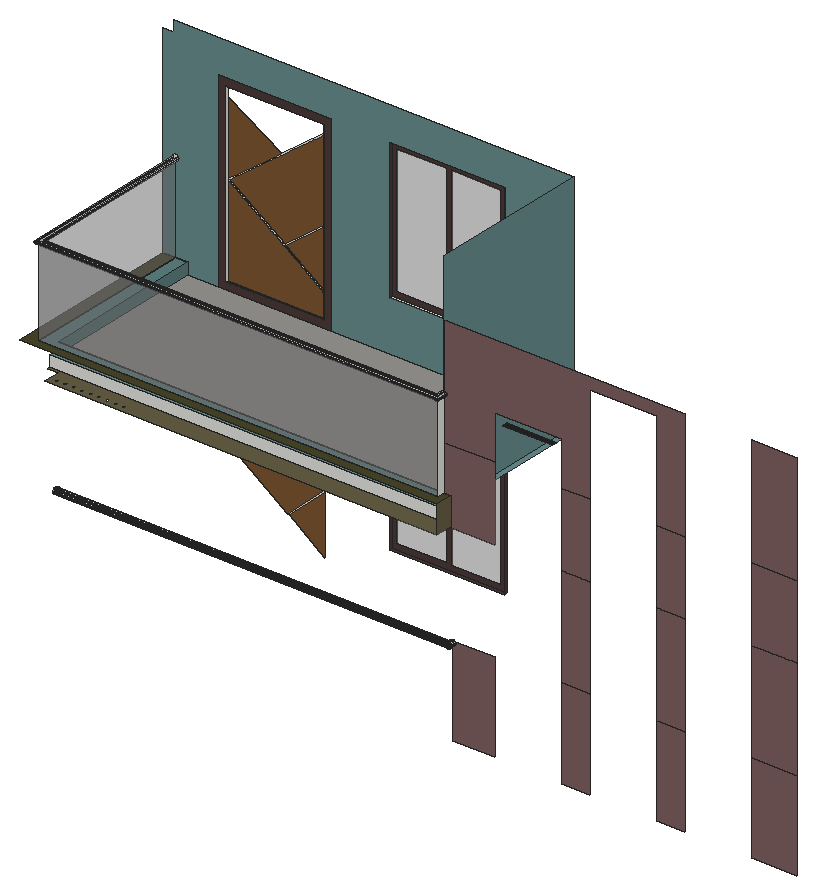
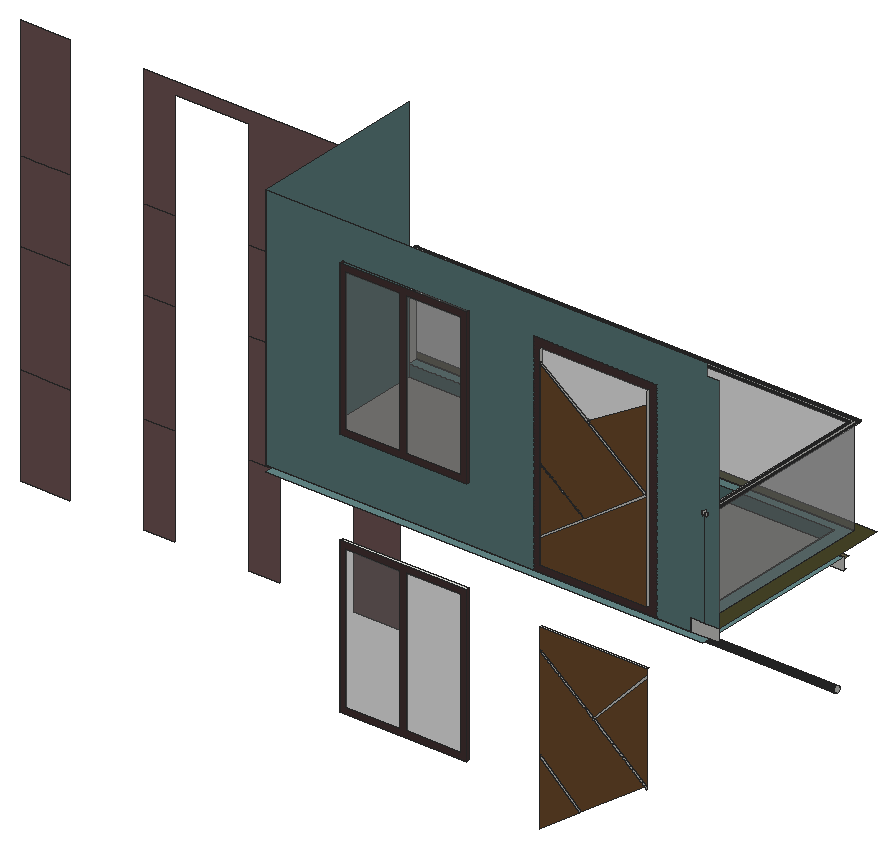
# SketchUp Ruby script. Lengths in inches.
U = 1.inch
M = Sketchup.active_model
def pt(a) = Geom::Point3d.new(a.map { |v| v * U })
def face(e, loops, mat)
  f = e.add_face(loops[0].map { |a| pt(a) })
  loops[1..].each { |l| e.add_face(l.map { |a| pt(a) }).erase! }
  f.material = f.back_material = mat if mat
  f
end
# faces: each face lists its corners as indices into pts; further lists are holes
def faces(e, pts, list, mat = nil) = list.each { |f| face(e, (f[0].is_a?(Array) ? f : [f]).map { |l| l.map { |i| pts[i] } }, mat) }
# xy, xz, yz: faces in a plane at the given z, y or x. An outline is a flat list of corners, or four numbers for a rectangle; further outlines are holes
def ring(l) = l.size == 4 ? [[l[0], l[1]], [l[2], l[1]], [l[2], l[3]], [l[0], l[3]]] : l.each_slice(2).to_a
def flat(e, list, mat, &to3) = list.each { |f| face(e, (f[0].is_a?(Array) ? f : [f]).map { |l| ring(l).map { |u, v| to3.(u, v) } }, mat) }
def xy(e, z, list, mat = nil) = flat(e, list, mat) { |x, y| [x, y, z] }
def xz(e, y, list, mat = nil) = flat(e, list, mat) { |x, z| [x, y, z] }
def yz(e, x, list, mat = nil) = flat(e, list, mat) { |y, z| [x, y, z] }
def lines(e, pts, list) = list.each { |a, b| e.add_line(pt(pts[a]), pt(pts[b])) }
# prism: a flat outline (further loops are holes) pulled along v
def prism(e, loops, v, mat = nil)
  f = face(e, loops, mat); d = Geom::Vector3d.new(v.map { |x| x * U })
  f.pushpull(f.normal.samedirection?(d) ? d.length : -d.length)
end
def box(e, o, s, mat = nil) = prism(e, [[o, [o[0] + s[0], o[1], o[2]], [o[0] + s[0], o[1] + s[1], o[2]], [o[0], o[1] + s[1], o[2]]]], [0, 0, s[2]], mat)
def at(x, y, z, deg = 0) = Geom::Transformation.translation(pt([x, y, z])) * Geom::Transformation.rotation(ORIGIN, Z_AXIS, deg.degrees)
def axes(o, x, y, z) = Geom::Transformation.new([*x, 0, *y, 0, *z, 0, *pt(o).to_a, 1])
def part(name) = M.definitions.add(name)
# library, detail: a bought-in or finely detailed component or shape, given as its bounding box
def library(name, o, s) = part(name).tap { |d| box(d.entities, o, s) }
def detail(e, o, s) = box(e.add_group.entities, o, s)
def put(e, d, t, mat = nil) = e.add_instance(d, t).tap { |i| i.material = mat if mat }
def group(e, t, mat = nil) = e.add_group.tap { |g| g.transformation = t; g.material = mat if mat }.entities
root = M.entities
M.materials.add("[0057_DarkKhaki]").color = [71, 69, 40]
M.materials.add("[0089_PaleTurquoise]").color = [103, 140, 140]
M.materials.add("[0089_PaleTurquoise]2").color = [93, 127, 127]
M.materials.add("[0119_RosyBrown]").color = [127, 96, 96]
M.materials.add("[0119_RosyBrown]1").color = [76, 58, 58]
M.materials.add("[0136_Charcoal]").color = [35, 35, 35]
M.materials.add("[Granite Light Gray]").color = [149, 148, 144]
M.materials.add("[Translucent Glass Gray]").color = [130, 130, 130]
M.materials["[Translucent Glass Gray]"].alpha = 0.5
M.materials.add("[Translucent Glass Gray]1").color = [128, 128, 128]
M.materials["[Translucent Glass Gray]1"].alpha = 0.5
M.materials.add("[Wood Floor]").color = [124, 84, 49]
M.materials.add("[Wood Lumber ButtJoined]").color = [102, 94, 69]
xy(root,619.5,[[726,546,973.25,552]],"[0119_RosyBrown]1")
xy(root,903.9,[[375.6,546,584.4,551]])
xy(root,919.5,[[726,546,973.25,552]])
xy(root,960,[[[294,162,294,198,270,198,270,204,1122,204,1122,198,1135.625,198,1135.625,162],[308.5625,171.77,309.6,171.91,310.5625,172.31,311.39,172.94,312.03,173.77,312.43,174.74,312.5625,175.77,312.43,176.81,312.03,177.77,311.39,178.6,310.5625,179.24,309.6,179.64,308.5625,179.77,307.53,179.64,306.5625,179.24,305.73,178.6,305.1,177.77,304.7,176.81,304.5625,175.77,304.7,174.74,305.1,173.77,305.73,172.94,306.5625,172.31,307.53,171.91],[326.5625,171.77,327.6,171.91,328.5625,172.31,329.39,172.94,330.03,173.77,330.43,174.74,330.5625,175.77,330.43,176.81,330.03,177.77,329.39,178.6,328.5625,179.24,327.6,179.64,326.5625,179.77,325.53,179.64,324.5625,179.24,323.73,178.6,323.1,177.77,322.7,176.81,322.5625,175.77,322.7,174.74,323.1,173.77,323.73,172.94,324.5625,172.31,325.53,171.91],[344.5625,171.77,345.6,171.91,346.5625,172.31,347.39,172.94,348.03,173.77,348.43,174.74,348.5625,175.77,348.43,176.81,348.03,177.77,347.39,178.6,346.5625,179.24,345.6,179.64,344.5625,179.77,343.53,179.64,342.5625,179.24,341.73,178.6,341.1,177.77,340.7,176.81,340.5625,175.77,340.7,174.74,341.1,173.77,341.73,172.94,342.5625,172.31,343.53,171.91],[362.5625,171.77,363.6,171.91,364.5625,172.31,365.39,172.94,366.03,173.77,366.43,174.74,366.5625,175.77,366.43,176.81,366.03,177.77,365.39,178.6,364.5625,179.24,363.6,179.64,362.5625,179.77,361.53,179.64,360.5625,179.24,359.73,178.6,359.1,177.77,358.7,176.81,358.5625,175.77,358.7,174.74,359.1,173.77,359.73,172.94,360.5625,172.31,361.53,171.91],[380.5625,171.77,381.6,171.91,382.5625,172.31,383.39,172.94,384.03,173.77,384.43,174.74,384.5625,175.77,384.43,176.81,384.03,177.77,383.39,178.6,382.5625,179.24,381.6,179.64,380.5625,179.77,379.53,179.64,378.5625,179.24,377.73,178.6,377.1,177.77,376.7,176.81,376.5625,175.77,376.7,174.74,377.1,173.77,377.73,172.94,378.5625,172.31,379.53,171.91],[398.5625,171.77,399.6,171.91,400.5625,172.31,401.39,172.94,402.03,173.77,402.43,174.74,402.5625,175.77,402.43,176.81,402.03,177.77,401.39,178.6,400.5625,179.24,399.6,179.64,398.5625,179.77,397.53,179.64,396.5625,179.24,395.73,178.6,395.1,177.77,394.7,176.81,394.5625,175.77,394.7,174.74,395.1,173.77,395.73,172.94,396.5625,172.31,397.53,171.91],[416.5625,171.77,417.6,171.91,418.5625,172.31,419.39,172.94,420.03,173.77,420.43,174.74,420.5625,175.77,420.43,176.81,420.03,177.77,419.39,178.6,418.5625,179.24,417.6,179.64,416.5625,179.77,415.53,179.64,414.5625,179.24,413.73,178.6,413.1,177.77,412.7,176.81,412.5625,175.77,412.7,174.74,413.1,173.77,413.73,172.94,414.5625,172.31,415.53,171.91],[434.5625,171.77,435.6,171.91,436.5625,172.31,437.39,172.94,438.03,173.77,438.43,174.74,438.5625,175.77,438.43,176.81,438.03,177.77,437.39,178.6,436.5625,179.24,435.6,179.64,434.5625,179.77,433.53,179.64,432.5625,179.24,431.73,178.6,431.1,177.77,430.7,176.81,430.5625,175.77,430.7,174.74,431.1,173.77,431.73,172.94,432.5625,172.31,433.53,171.91],[452.5625,171.77,453.6,171.91,454.5625,172.31,455.39,172.94,456.03,173.77,456.43,174.74,456.5625,175.77,456.43,176.81,456.03,177.77,455.39,178.6,454.5625,179.24,453.6,179.64,452.5625,179.77,451.53,179.64,450.5625,179.24,449.73,178.6,449.1,177.77,448.7,176.81,448.5625,175.77,448.7,174.74,449.1,173.77,449.73,172.94,450.5625,172.31,451.53,171.91]]],"[Wood Lumber ButtJoined]")
xy(root,984,[[382.18,289.15,379.08,289.56,376.18,290.76,373.7,292.66,371.79,295.15,370.59,298.04,370.18,301.15,370.59,304.26,371.79,307.15,373.7,309.63,376.18,311.54,379.08,312.74,382.18,313.15,385.29,312.74,388.18,311.54,390.67,309.63,392.58,307.15,393.77,304.26,394.18,301.15,393.77,298.04,392.58,295.15,390.67,292.66,388.18,290.76,385.29,289.56],[706.18,289.15,703.08,289.56,700.18,290.76,697.7,292.66,695.79,295.15,694.59,298.04,694.18,301.15,694.59,304.26,695.79,307.15,697.7,309.63,700.18,311.54,703.08,312.74,706.18,313.15,709.29,312.74,712.18,311.54,714.67,309.63,716.58,307.15,717.77,304.26,718.18,301.15,717.77,298.04,716.58,295.15,714.67,292.66,712.18,290.76,709.29,289.56],[1030.18,289.15,1027.08,289.56,1024.18,290.76,1021.7,292.66,1019.79,295.15,1018.59,298.04,1018.18,301.15,1018.59,304.26,1019.79,307.15,1021.7,309.63,1024.18,311.54,1027.08,312.74,1030.18,313.15,1033.29,312.74,1036.18,311.54,1038.67,309.63,1040.58,307.15,1041.77,304.26,1042.18,301.15,1041.77,298.04,1040.58,295.15,1038.67,292.66,1036.18,290.76,1033.29,289.56],[382.18,409.15,379.08,409.56,376.18,410.76,373.7,412.66,371.79,415.15,370.59,418.04,370.18,421.15,370.59,424.26,371.79,427.15,373.7,429.63,376.18,431.54,379.08,432.74,382.18,433.15,385.29,432.74,388.18,431.54,390.67,429.63,392.58,427.15,393.77,424.26,394.18,421.15,393.77,418.04,392.58,415.15,390.67,412.66,388.18,410.76,385.29,409.56],[706.18,409.15,703.08,409.56,700.18,410.76,697.7,412.66,695.79,415.15,694.59,418.04,694.18,421.15,694.59,424.26,695.79,427.15,697.7,429.63,700.18,431.54,703.08,432.74,706.18,433.15,709.29,432.74,712.18,431.54,714.67,429.63,716.58,427.15,717.77,424.26,718.18,421.15,717.77,418.04,716.58,415.15,714.67,412.66,712.18,410.76,709.29,409.56],
  [1030.18,409.15,1027.08,409.56,1024.18,410.76,1021.7,412.66,1019.79,415.15,1018.59,418.04,1018.18,421.15,1018.59,424.26,1019.79,427.15,1021.7,429.63,1024.18,431.54,1027.08,432.74,1030.18,433.15,1033.29,432.74,1036.18,431.54,1038.67,429.63,1040.58,427.15,1041.77,424.26,1042.18,421.15,1041.77,418.04,1040.58,415.15,1038.67,412.66,1036.18,410.76,1033.29,409.56]])
xy(root,984,[[[270,204,1122,546],[382.18,409.15,385.29,409.56,388.18,410.76,390.67,412.66,392.58,415.15,393.77,418.04,394.18,421.15,393.77,424.26,392.58,427.15,390.67,429.63,388.18,431.54,385.29,432.74,382.18,433.15,379.08,432.74,376.18,431.54,373.7,429.63,371.79,427.15,370.59,424.26,370.18,421.15,370.59,418.04,371.79,415.15,373.7,412.66,376.18,410.76,379.08,409.56],[382.18,289.15,385.29,289.56,388.18,290.76,390.67,292.66,392.58,295.15,393.77,298.04,394.18,301.15,393.77,304.26,392.58,307.15,390.67,309.63,388.18,311.54,385.29,312.74,382.18,313.15,379.08,312.74,376.18,311.54,373.7,309.63,371.79,307.15,370.59,304.26,370.18,301.15,370.59,298.04,371.79,295.15,373.7,292.66,376.18,290.76,379.08,289.56],[706.18,409.15,709.29,409.56,712.18,410.76,714.67,412.66,716.58,415.15,717.77,418.04,718.18,421.15,717.77,424.26,716.58,427.15,714.67,429.63,712.18,431.54,709.29,432.74,706.18,433.15,703.08,432.74,700.18,431.54,697.7,429.63,695.79,427.15,694.59,424.26,694.18,421.15,694.59,418.04,695.79,415.15,697.7,412.66,700.18,410.76,703.08,409.56],[1030.18,409.15,1033.29,409.56,1036.18,410.76,1038.67,412.66,1040.58,415.15,1041.77,418.04,1042.18,421.15,1041.77,424.26,1040.58,427.15,1038.67,429.63,1036.18,431.54,1033.29,432.74,1030.18,433.15,1027.08,432.74,1024.18,431.54,1021.7,429.63,1019.79,427.15,1018.59,424.26,1018.18,421.15,1018.59,418.04,1019.79,415.15,1021.7,412.66,1024.18,410.76,1027.08,409.56],[706.18,289.15,709.29,289.56,712.18,290.76,714.67,292.66,716.58,295.15,717.77,298.04,718.18,301.15,717.77,304.26,716.58,307.15,714.67,309.63,712.18,311.54,709.29,312.74,706.18,313.15,703.08,312.74,700.18,311.54,697.7,309.63,695.79,307.15,694.59,304.26,694.18,301.15,694.59,298.04,695.79,295.15,697.7,292.66,700.18,290.76,703.08,289.56],[1030.18,289.15,1033.29,289.56,1036.18,290.76,1038.67,292.66,1040.58,295.15,1041.77,298.04,1042.18,301.15,1041.77,304.26,1040.58,307.15,1038.67,309.63,1036.18,311.54,1033.29,312.74,1030.18,313.15,1027.08,312.74,1024.18,311.54,1021.7,309.63,1019.79,307.15,1018.59,304.26,1018.18,301.15,1018.59,298.04,1019.79,295.15,1021.7,292.66,1024.18,290.76,1027.08,289.56]]],"[0089_PaleTurquoise]")
xy(root,996,[[294,198,1122,546]],"[Granite Light Gray]")
xy(root,1011.6,[[375.6,546,584.4,551]])
xy(root,1020,[[240,162,1135.625,162,1135.625,198,1122,198,1122,180,267,180,267,546,240,546]],"[0057_DarkKhaki]")
xy(root,1020,[[267,180,1122,180,1122,198,294,198,294,546,267,546]],"[0089_PaleTurquoise]2")
xy(root,1104,[[726,546,973.25,552]])
xy(root,1194,[[1248,198,1356,208]],"[0136_Charcoal]")
xz(root,180,[[267,1206,1122,1212]])
xz(root,180,[[267,1020,1122,1206]],"[Translucent Glass Gray]")
xz(root,198,[[1122,960,1135.625,984],[1122,996,1135.625,1020]])
xz(root,198,[[294,996,1122,1020]],"[0089_PaleTurquoise]2")
xz(root,198,[[1140.5,549.1875,1230,549.1875,1230,742.375,1144.72,742.27,1145.68,741.03,1146.29,739.58,1146.5,738.03,1146.3,736.48,1145.71,735.03,1144.77,733.78,1143.53,732.82,1142.08,732.21,1140.53,732,1140.5,732],[1374,549.1875,1434,742.375],[1578,549.1875,1638,742.375],[1782,549.1875,1879.2,742.375],[1374,742.375,1434,958.375],
  [1578,742.375,1638,958.375],[1782,742.375,1879.2,958.375],[1122,958.375,1230,958.375,1230,1117.25,1122,1117.25,1122,1020,1135.625,1020,1135.625,960,1122,960],[1374,958.375,1434,1117.25],[1578,958.375,1638,1117.25],
  [1782,958.375,1879.2,1117.25],[1122,1117.25,1230,1117.25,1230,1212,1374,1212,1374,1117.25,1434,1117.25,1434,1328.4375,1578,1328.4375,1578,1117.25,1638,1117.25,1638,1353.5,1122,1353.5,1122,1218,1123.55,1217.8,1125,1217.2,1126.24,1216.24,1127.2,1215,1127.8,1213.55,1128,1212,1127.8,1210.45,1127.2,1209,1126.24,1207.76,1125,1206.8,1123.55,1206.2,1122,1206],[1782,1117.25,1879.2,1353.5]],"[0119_RosyBrown]")
xz(root,204,[[270,960,1122,984]])
xz(root,546,[[240,996,294,1020],[267,1206,265.45,1206.2,264,1206.8,262.76,1207.76,261.8,1209,261.2,1210.45,261,1212,261.2,1213.55,261.8,1215,262.76,1216.24,264,1217.2,265.45,1217.8,267,1218,268.55,1217.8,270,1217.2,271.24,1216.24,272.2,1215,272.8,1213.55,273,1212,272.8,1210.45,272.2,1209,271.24,1207.76,270,1206.8,268.55,1206.2]])
xz(root,546,[[[294,996,360,996,360,1404,600,1404,600,996,1122,996,1122,1476,264,1476,264,1452,240,1452,240,1020,294,1020],[726,1104,973.25,1404],[267,1206,265.45,1206.2,264,1206.8,262.76,1207.76,261.8,1209,261.2,1210.45,261,1212,261.2,1213.55,261.8,1215,262.76,1216.24,264,1217.2,265.45,1217.8,267,1218,268.55,1217.8,270,1217.2,271.24,1216.24,272.2,1215,272.8,1213.55,273,1212,272.8,1210.45,272.2,1209,271.24,1207.76,270,1206.8,268.55,1206.2]]],"[0089_PaleTurquoise]")
xz(root,546,[[[360,996,600,1404],[375.6,1011.6,584.4,1388.4]]],"[0119_RosyBrown]1")
xz(root,551,[[507.28,606.22,584.4,676.57,584.4,681.98,503.9375,608.57],[375.6,692.98,379.5,696.14,584.4,861.91,584.4,866.29,480,782.61,477.54,780.63,375.6,698.92],[477.54,780.63,480,782.61,375.6,891.82,375.6,886.45],[584.4,1059.79,584.4,1063.17,499.53,1122.23,496.97,1124.01,379.36,1205.83,376.63,1203.72],[499.53,1122.23,584.4,1188.79,584.4,1192.53,496.97,1124.01],
  [376.63,1203.72,379.36,1205.83,584.4,1364.5,584.4,1368.29,493.62,1298.62,490.26,1296.05,375.6,1208.05,375.6,1204.43]])
xz(root,551,[[584.4,551.94,584.4,676.57,507.28,606.22],[503.9375,608.57,584.4,681.98,584.4,861.91,379.5,696.14],[375.6,698.92,477.54,780.63,375.6,886.45],[480,782.61,584.4,866.29,584.4,903.9,375.6,903.9,375.6,891.82],[375.6,1011.6,584.4,1011.6,584.4,1059.79,376.63,1203.72,375.6,1204.43],
  [584.4,1063.17,584.4,1188.79,499.53,1122.23],[496.97,1124.01,584.4,1192.53,584.4,1364.5,379.36,1205.83],[375.6,1208.05,490.26,1296.05,375.6,1364.68]],"[Wood Floor]")
xz(root,552,[[[726,619.5,973.25,919.5],[738,631.5,843.625,907.5],[855.625,631.5,961.25,907.5]],[[726,1104,973.25,1404],[855.625,1116,961.25,1392],[738,1116,843.625,1392]]],"[0119_RosyBrown]1")
xz(root,552,[[738,631.5,843.625,907.5],[855.625,631.5,961.25,907.5],[738,1116,843.625,1392],[855.625,1116,961.25,1392]],"[Translucent Glass Gray]1")
yz(root,267,[[180,1206,546,1212]])
yz(root,267,[[180,1020,546,1206]],"[Translucent Glass Gray]")
yz(root,294,[[189.51,732,187.96,732.21,186.52,732.82,185.28,733.78,184.33,735.03,183.74,736.48,183.55,738.03,183.76,739.58,184.37,741.03,185.33,742.27,186.57,743.21,188.02,743.8,189.58,744,191.13,743.79,192.57,743.18,193.8125,742.22,194.76,740.97,195.35,739.52,195.55,737.97,195.33,736.42,194.72,734.97,193.76,733.73,192.52,732.79,191.07,732.2,189.55,732]])
yz(root,294,[[198,996,546,1020]],"[0089_PaleTurquoise]2")
yz(root,375.6,[[546,1011.6,551,1388.4]])
yz(root,584.4,[[546,1011.6,551,1388.4]])
yz(root,726,[[546,619.5,552,919.5],[546,1104,552,1404]],"[0119_RosyBrown]1")
yz(root,973.25,[[546,619.5,552,919.5],[546,1104,552,1404]],"[0119_RosyBrown]1")
yz(root,1122,[[198,960,204,984],[180,1020,198,1206],[180,1206,198,1212]])
yz(root,1122,[[198,996,546,1476]],"[0089_PaleTurquoise]")
yz(root,1135.625,[[162,960,198,1020]],"[Wood Lumber ButtJoined]")
p = [[294,187.96,732.21],[294,189.51,732],[1140.53,189.51,732],[1142.08,187.96,732.21],[1140.53,198,732],[1142.08,198,732.21],
  [294,189.55,732],[294,191.07,732.2],[1138.98,191.07,732.2],[1140.5,189.55,732],[1138.98,198,732.2],[1140.5,198,732],
  [294,186.52,732.82],[1143.53,186.52,732.82],[1143.53,198,732.82],[294,192.52,732.79],[1137.53,192.52,732.79],[1137.53,198,732.79],
  [294,185.28,733.78],[1144.77,185.28,733.78],[1144.77,198,733.78],[294,193.76,733.73],[1136.28,193.76,733.73],[1136.28,198,733.73],
  [294,194.72,734.97],[1135.32,194.72,734.97],[1135.32,198,734.97],[294,184.33,735.03],[1145.71,184.33,735.03],[1145.71,198,735.03],
  [294,183.74,736.48],[1146.3,183.74,736.48],[1146.3,198,736.48],[294,195.33,736.42],[1134.71,195.33,736.42],[1134.71,198,736.42],
  [294,195.55,737.97],[1134.5,195.55,737.97],[1134.5,198,737.97],[294,183.55,738.03],[1146.5,183.55,738.03],[1146.5,198,738.03],
  [294,183.76,739.58],[1146.29,183.76,739.58],[1146.29,198,739.58],[294,195.35,739.52],[1134.7,195.35,739.52],[1134.7,198,739.52],
  [294,194.76,740.97],[1135.29,194.76,740.97],[1135.29,198,740.97],[294,184.37,741.03],[1145.68,184.37,741.03],[1145.68,198,741.03],
  [294,185.33,742.27],[1144.72,185.33,742.27],[1144.72,198,742.27],[294,193.8125,742.22],[1136.23,193.8125,742.22],[1136.23,198,742.22],
  [294,192.57,743.18],[1137.47,192.57,743.18],[1137.47,198,743.18],[294,186.57,743.21],[1143.47,186.57,743.21],[1143.47,198,743.21],
  [294,188.02,743.8],[1142.02,188.02,743.8],[1142.02,198,743.8],[294,191.13,743.79],[1138.92,191.13,743.79],[1138.92,198,743.79],
  [294,189.58,744],[1140.47,189.58,744],[1140.47,198,744],[265.45,178.45,1206.2],[267,180,1206],[1122,180,1206],
  [1123.55,178.45,1206.2],[265.45,546,1206.2],[267,546,1206],[1122,198,1206],[1123.55,198,1206.2],[268.55,181.55,1206.2],
  [1120.45,181.55,1206.2],[268.55,546,1206.2],[1120.45,198,1206.2],[264,177,1206.8],[1125,177,1206.8],[264,546,1206.8],
  [1125,198,1206.8],[270,183,1206.8],[1119,183,1206.8],[270,546,1206.8],[1119,198,1206.8],[262.76,175.76,1207.76],
  [1126.24,175.76,1207.76],[262.76,546,1207.76],[1126.24,198,1207.76],[271.24,184.24,1207.76],[1117.76,184.24,1207.76],[271.24,546,1207.76],
  [1117.76,198,1207.76],[261.8,174.8,1209],[1127.2,174.8,1209],[261.8,546,1209],[1127.2,198,1209],[272.2,185.2,1209],
  [1116.8,185.2,1209],[272.2,546,1209],[1116.8,198,1209],[261.2,174.2,1210.45],[1127.8,174.2,1210.45],[261.2,546,1210.45],
  [1127.8,198,1210.45],[272.8,185.8,1210.45],[1116.2,185.8,1210.45],[272.8,546,1210.45],[1116.2,198,1210.45],[261,174,1212],
  [1128,174,1212],[261,546,1212],[1128,198,1212],[273,186,1212],[1116,186,1212],[273,546,1212],
  [1116,198,1212],[261.2,174.2,1213.55],[1127.8,174.2,1213.55],[261.2,546,1213.55],[1127.8,198,1213.55],[272.8,185.8,1213.55],
  [1116.2,185.8,1213.55],[272.8,546,1213.55],[1116.2,198,1213.55]]
faces(root,p,[[0,1,2,3],[3,2,4,5],[1,6,7,8,9,2],[9,8,10,11,4,2],[12,0,3,13],[13,3,5,14],[7,15,16,8],[8,16,17,10],
  [18,12,13,19],[19,13,14,20],[15,21,22,16],[16,22,23,17],[21,24,25,22],[22,25,26,23],[27,18,19,28],[28,19,20,29],
  [30,27,28,31],[31,28,29,32],[24,33,34,25],[25,34,35,26],[33,36,37,34],[34,37,38,35],[39,30,31,40],[40,31,32,41],
  [42,39,40,43],[43,40,41,44],[36,45,46,37],[37,46,47,38],[45,48,49,46],[46,49,50,47],[51,42,43,52],[52,43,44,53],
  [54,51,52,55],[55,52,53,56],[48,57,58,49],[49,58,59,50],[57,60,61,58],[58,61,62,59],[63,54,55,64],[64,55,56,65],
  [66,63,64,67],[67,64,65,68],[60,69,70,61],[61,70,71,62],[72,66,67,73],[73,67,68,74],[69,72,73,70],[70,73,74,71],
  [75,76,77,78],[79,80,76,75],[78,77,81,82],[76,83,84,77],[80,85,83,76],[77,84,86,81],[87,75,78,88],[89,79,75,87],
  [88,78,82,90],[83,91,92,84],[85,93,91,83],[84,92,94,86],[95,87,88,96],[97,89,87,95],[96,88,90,98],[91,99,100,92],
  [93,101,99,91],[92,100,102,94],[103,95,96,104],[105,97,95,103],[104,96,98,106],[99,107,108,100],[101,109,107,99],[100,108,110,102],
  [111,103,104,112],[113,105,103,111],[112,104,106,114],[107,115,116,108],[109,117,115,107],[108,116,118,110],[119,111,112,120],[121,113,111,119],
  [120,112,114,122],[115,123,124,116],[117,125,123,115],[116,124,126,118],[127,119,120,128],[129,121,119,127],[128,120,122,130],[123,131,132,124],
  [125,133,131,123],[124,132,134,126]])
